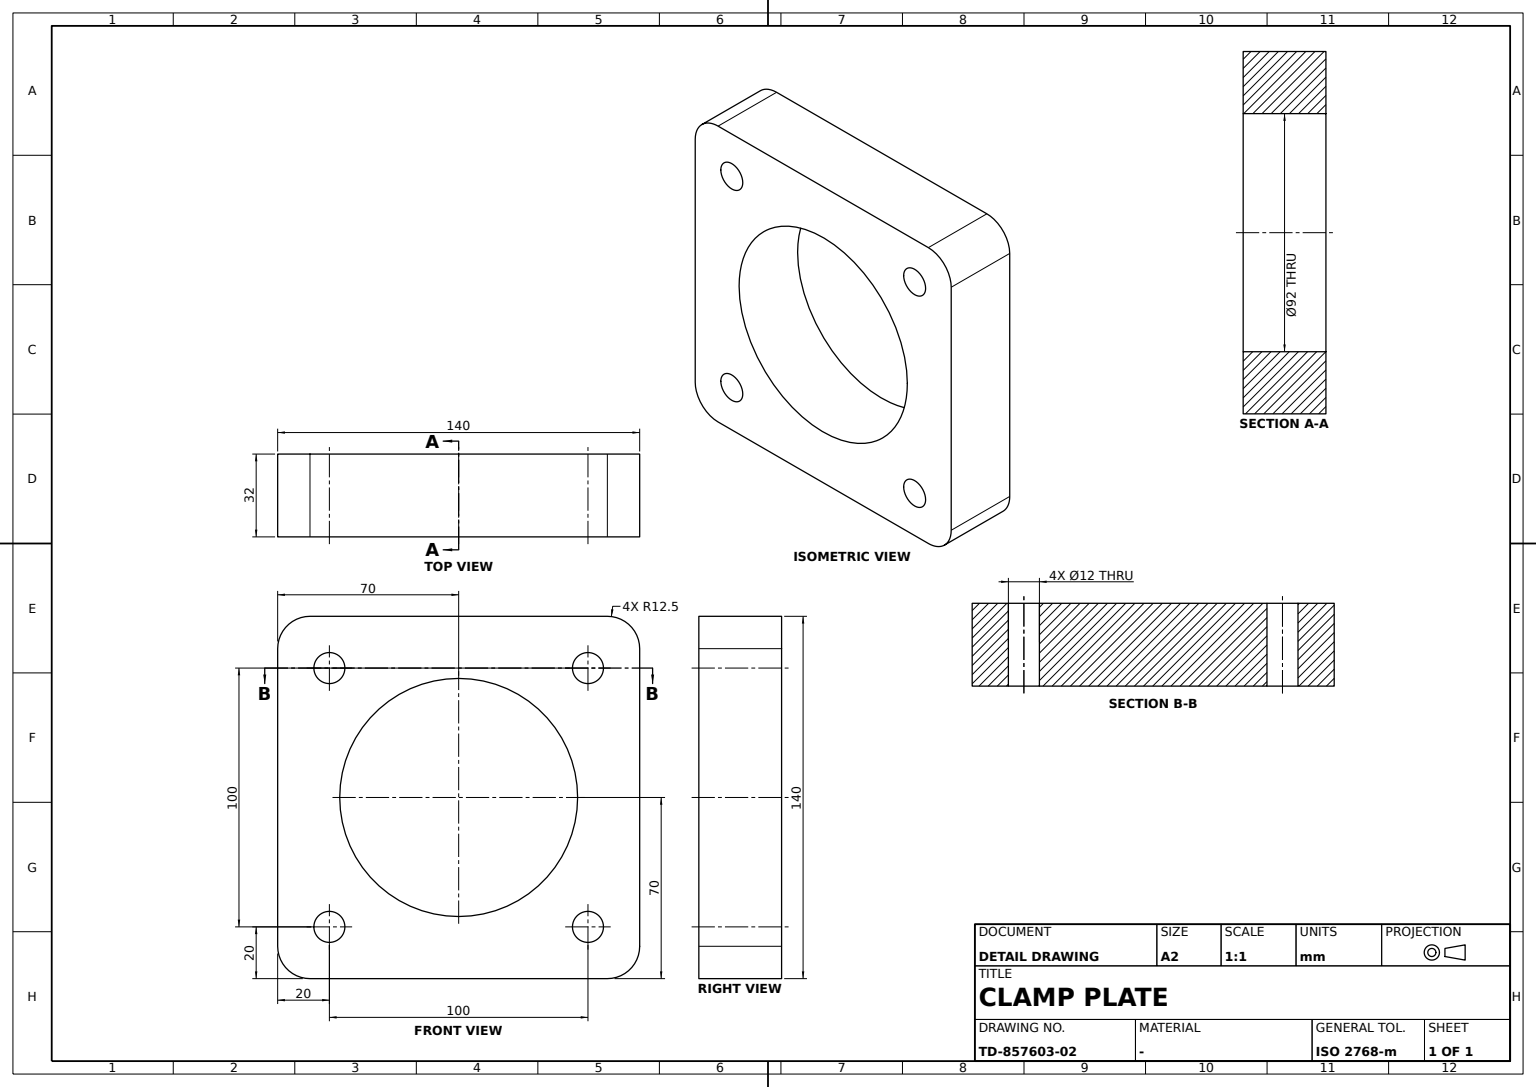
solid
v1 (132.5,-32,28)
v2 (132.5,-32,0)
e1 v1 v2 LINE
v3 (132.5,-60,28)
e2 v1 v3 CIRCLE(AX(P(132.5,-46,28),D(0,0,1),D(1,0,0)),14)
v4 (132.5,-60,0)
e3 v3 v4 LINE
e4 v2 v4 CIRCLE(AX(P(132.5,-46,0),D(0,0,1),D(1,0,0)),14)
face CYL(AX(P(132.5,-46,28),D(0,0,-1),D(1,0,0)),14) rev [-e1 e2 e3 -e4]
v5 (152.5,-89,28)
v6 (152.5,-76.5,28)
e5 v5 v6 LINE
v7 (140,-89,28)
e6 v7 v5 LINE
e7 v6 v7 CIRCLE(AX(P(140,-76.5,28),D(0,0,-1),D(1,0,0)),12.5)
face PLANE(AX(P(0,0,28),D(0,0,1),D(1,0,0))) rev [-e5 -e6 -e7]
v8 (152.5,89,28)
v9 (152.5,89,56)
e8 v8 v9 LINE
v10 (140,89,28)
e9 v8 v10 LINE
v11 (140,89,0)
e10 v11 v10 LINE
v12 (-140,89,0)
e11 v11 v12 LINE
v13 (-140,89,28)
e12 v12 v13 LINE
v14 (-152.5,89,28)
e13 v13 v14 LINE
v15 (-152.5,89,56)
e14 v14 v15 LINE
e15 v9 v15 LINE
face PLANE(AX(P(-152.5,89,0),D(0,-1,0),D(1,0,0))) rev [-e8 e9 -e10 e11 e12 e13 e14 -e15]
v16 (9.365911,-50,0)
v17 (-2.634089,-50,0)
e16 v16 v17 CIRCLE(AX(P(3.365911,-50,0),D(0,0,-1),D(1,0,0)),6)
e17 v17 v16 CIRCLE(AX(P(3.365911,-50,0),D(0,0,-1),D(1,0,0)),6)
face PLANE(AX(P(0,0,0),D(0,0,1),D(1,0,0))) rev [e16 e17]
v18 (-152.5,76.5,28)
e18 v18 v13 CIRCLE(AX(P(-140,76.5,28),D(0,0,-1),D(1,0,0)),12.5)
v19 (-152.5,76.5,0)
e19 v12 v19 CIRCLE(AX(P(-140,76.5,0),D(0,0,1),D(1,0,0)),12.5)
e20 v19 v18 LINE
face CYL(AX(P(-140,76.5,14),D(0,0,-1),D(-1,0,0)),12.5) [e18 -e12 e19 e20]
v20 (152.5,-32,28)
v21 (152.5,-32,0)
e21 v20 v21 LINE
e22 v20 v1 LINE
e23 v21 v2 LINE
face PLANE(AX(P(152.5,-32,28),D(0,1,0),D(1,0,0))) rev [-e21 e22 e1 -e23]
v22 (152.5,-76.5,0)
e24 v22 v6 LINE
v23 (140,-89,0)
e25 v23 v7 LINE
e26 v23 v22 CIRCLE(AX(P(140,-76.5,0),D(0,0,1),D(1,0,0)),12.5)
face CYL(AX(P(140,-76.5,14),D(0,0,-1),D(1,0,0)),12.5) [e24 e7 -e25 e26]
v24 (-2.634089,50,0)
v25 (-2.634089,50,-32)
e27 v24 v25 LINE
v26 (9.365911,50,0)
e28 v26 v24 CIRCLE(AX(P(3.365911,50,0),D(0,0,-1),D(1,0,0)),6)
v27 (9.365911,50,-32)
e29 v26 v27 LINE
e30 v27 v25 CIRCLE(AX(P(3.365911,50,-32),D(0,0,-1),D(1,0,0)),6)
face CYL(AX(P(3.365911,50,-16),D(0,0,1),D(1,0,0)),6) rev [-e27 -e28 e29 e30]
v28 (-2.634089,-50,-32)
v29 (9.365911,-50,-32)
e31 v28 v29 CIRCLE(AX(P(3.365911,-50,-32),D(0,0,-1),D(1,0,0)),6)
e32 v16 v29 LINE
e33 v17 v28 LINE
face CYL(AX(P(3.365911,-50,-16),D(0,0,1),D(1,0,0)),6) rev [e31 -e32 -e17 e33]
v30 (-90.634089,50,0)
v31 (-90.634089,50,-32)
e34 v30 v31 LINE
v32 (-102.634089,50,0)
e35 v32 v30 CIRCLE(AX(P(-96.634089,50,0),D(0,0,-1),D(1,0,0)),6)
v33 (-102.634089,50,-32)
e36 v32 v33 LINE
e37 v33 v31 CIRCLE(AX(P(-96.634089,50,-32),D(0,0,-1),D(1,0,0)),6)
face CYL(AX(P(-96.634089,50,-16),D(0,0,1),D(1,0,0)),6) rev [-e34 -e35 e36 e37]
v34 (-116.634089,57.5,0)
v35 (-116.634089,57.5,-32)
e38 v34 v35 LINE
v36 (-116.634089,-57.5,-32)
e39 v36 v35 LINE
v37 (-116.634089,-57.5,0)
e40 v37 v36 LINE
e41 v37 v34 LINE
face PLANE(AX(P(-116.634089,-70,0),D(-1,0,0),D(0,1,0))) [e38 -e39 -e40 e41]
v38 (-102.634089,-50,0)
v39 (-90.634089,-50,0)
e42 v38 v39 CIRCLE(AX(P(-96.634089,-50,0),D(0,0,-1),D(1,0,0)),6)
v40 (-102.634089,-50,-32)
e43 v38 v40 LINE
v41 (-90.634089,-50,-32)
e44 v40 v41 CIRCLE(AX(P(-96.634089,-50,-32),D(0,0,-1),D(1,0,0)),6)
e45 v39 v41 LINE
face CYL(AX(P(-96.634089,-50,-16),D(0,0,1),D(1,0,0)),6) rev [-e42 e43 e44 -e45]
v42 (23.365911,-57.5,0)
v43 (10.865911,-70,0)
e46 v42 v43 CIRCLE(AX(P(10.865911,-57.5,0),D(0,0,-1),D(1,0,0)),12.5)
v44 (10.865911,-70,-32)
e47 v43 v44 LINE
v45 (23.365911,-57.5,-32)
e48 v44 v45 CIRCLE(AX(P(10.865911,-57.5,-32),D(0,0,1),D(1,0,0)),12.5)
e49 v42 v45 LINE
face CYL(AX(P(10.865911,-57.5,-16),D(0,0,1),D(0,-1,0)),12.5) [e46 e47 e48 -e49]
v46 (-132.5,32,28)
v47 (-118.5,46,28)
e50 v46 v47 CIRCLE(AX(P(-132.5,46,28),D(0,0,1),D(1,0,0)),14)
v48 (-152.5,32,28)
e51 v48 v46 LINE
v49 (-152.5,60,28)
e52 v49 v48 LINE
v50 (-132.5,60,28)
e53 v49 v50 LINE
e54 v47 v50 CIRCLE(AX(P(-132.5,46,28),D(0,0,1),D(1,0,0)),14)
face PLANE(AX(P(0,0,28),D(0,0,1),D(1,0,0))) rev [-e50 -e51 -e52 e53 -e54]
v51 (-118.5,-46,0)
v52 (-132.5,-32,0)
e55 v51 v52 CIRCLE(AX(P(-132.5,-46,0),D(0,0,1),D(1,0,0)),14)
v53 (-118.5,-46,28)
e56 v53 v51 LINE
v54 (-132.5,-32,28)
e57 v53 v54 CIRCLE(AX(P(-132.5,-46,28),D(0,0,1),D(1,0,0)),14)
e58 v54 v52 LINE
face CYL(AX(P(-132.5,-46,28),D(0,0,-1),D(1,0,0)),14) rev [-e55 -e56 e57 e58]
v55 (-152.5,-32,28)
v56 (-152.5,-32,0)
e59 v55 v56 LINE
e60 v52 v56 LINE
e61 v55 v54 LINE
face PLANE(AX(P(152.5,-32,28),D(0,1,0),D(1,0,0))) rev [e59 -e60 -e58 -e61]
e62 v30 v32 CIRCLE(AX(P(-96.634089,50,0),D(0,0,-1),D(1,0,0)),6)
face PLANE(AX(P(0,0,0),D(0,0,1),D(1,0,0))) rev [e62 e35]
e63 v25 v27 CIRCLE(AX(P(3.365911,50,-32),D(0,0,-1),D(1,0,0)),6)
e64 v24 v26 CIRCLE(AX(P(3.365911,50,0),D(0,0,-1),D(1,0,0)),6)
face CYL(AX(P(3.365911,50,-16),D(0,0,1),D(1,0,0)),6) rev [e63 -e29 -e64 e27]
e65 v31 v33 CIRCLE(AX(P(-96.634089,50,-32),D(0,0,-1),D(1,0,0)),6)
face CYL(AX(P(-96.634089,50,-16),D(0,0,1),D(1,0,0)),6) rev [e65 -e36 -e62 e34]
v57 (23.365911,57.5,-32)
e66 v57 v45 LINE
v58 (23.365911,57.5,0)
e67 v58 v57 LINE
e68 v58 v42 LINE
face PLANE(AX(P(23.365911,70,0),D(1,0,0),D(0,-1,0))) [-e66 -e67 e68 e49]
e69 v39 v38 CIRCLE(AX(P(-96.634089,-50,0),D(0,0,-1),D(1,0,0)),6)
face PLANE(AX(P(0,0,0),D(0,0,1),D(1,0,0))) rev [e69 e42]
v59 (-118.5,46,0)
v60 (-132.5,60,0)
e70 v59 v60 CIRCLE(AX(P(-132.5,46,0),D(0,0,1),D(1,0,0)),14)
e71 v47 v59 LINE
e72 v50 v60 LINE
face CYL(AX(P(-132.5,46,28),D(0,0,-1),D(1,0,0)),14) rev [-e70 -e71 e54 e72]
v61 (132.5,58.059115,28)
v62 (132.5,58.059115,0)
e73 v61 v62 LINE
v63 (132.5,33.940885,28)
e74 v61 v63 CIRCLE(AX(P(132.5,46,28),D(0,0,1),D(1,0,0)),12.059115)
v64 (132.5,33.940885,0)
e75 v63 v64 LINE
e76 v62 v64 CIRCLE(AX(P(132.5,46,0),D(0,0,1),D(1,0,0)),12.059115)
face CYL(AX(P(132.5,46,20),D(0,0,-1),D(1,0,0)),12.059115) rev [-e73 e74 e75 -e76]
v65 (152.5,58.059115,0)
e77 v65 v62 LINE
v66 (152.5,58.059115,28)
e78 v66 v65 LINE
e79 v66 v61 LINE
face PLANE(AX(P(152.5,58.059115,20),D(0,1,0),D(1,0,0))) rev [-e77 -e78 e79 e73]
v67 (-140,-89,28)
v68 (-152.5,-76.5,28)
e80 v67 v68 CIRCLE(AX(P(-140,-76.5,28),D(0,0,-1),D(1,0,0)),12.5)
v69 (-152.5,-76.5,0)
e81 v69 v68 LINE
v70 (-140,-89,0)
e82 v69 v70 CIRCLE(AX(P(-140,-76.5,0),D(0,0,1),D(1,0,0)),12.5)
e83 v70 v67 LINE
face CYL(AX(P(-140,-76.5,14),D(0,0,-1),D(0,-1,0)),12.5) [e80 -e81 e82 e83]
e84 v14 v18 LINE
face PLANE(AX(P(0,0,28),D(0,0,1),D(1,0,0))) rev [-e84 -e13 -e18]
v71 (-152.5,-89,28)
e85 v71 v67 LINE
e86 v68 v71 LINE
face PLANE(AX(P(0,0,28),D(0,0,1),D(1,0,0))) rev [-e80 -e85 -e86]
v72 (-152.5,-89,56)
e87 v71 v72 LINE
e88 v15 v72 LINE
v73 (-152.5,60,0)
e89 v19 v73 LINE
e90 v49 v73 LINE
v74 (-152.5,32,0)
e91 v48 v74 LINE
e92 v74 v56 LINE
v75 (-152.5,-60,28)
e93 v55 v75 LINE
v76 (-152.5,-60,0)
e94 v75 v76 LINE
e95 v76 v69 LINE
face PLANE(AX(P(-152.5,89,0),D(-1,0,0),D(0,-1,0))) [e86 e87 -e88 -e14 e84 -e20 e89 -e90 e52 e91 e92 -e59 e93 e94 e95 e81]
v77 (-132.5,-60,0)
e96 v77 v51 CIRCLE(AX(P(-132.5,-46,0),D(0,0,1),D(1,0,0)),14)
v78 (-132.5,-60,28)
e97 v78 v77 LINE
e98 v78 v53 CIRCLE(AX(P(-132.5,-46,28),D(0,0,1),D(1,0,0)),14)
face CYL(AX(P(-132.5,-46,28),D(0,0,-1),D(1,0,0)),14) rev [-e96 -e97 e98 e56]
e99 v70 v23 LINE
v79 (152.5,-89,56)
e100 v5 v79 LINE
e101 v72 v79 LINE
face PLANE(AX(P(152.5,-89,0),D(0,1,0),D(-1,0,0))) rev [e99 e25 e6 e100 -e101 -e87 e85 -e83]
v80 (152.5,-60,28)
e102 v80 v20 LINE
e103 v80 v3 LINE
face PLANE(AX(P(0,0,28),D(0,0,1),D(1,0,0))) rev [-e2 -e22 -e102 e103]
e104 v75 v78 LINE
face PLANE(AX(P(0,0,28),D(0,0,1),D(1,0,0))) rev [-e93 e61 -e57 -e98 -e104]
e105 v79 v9 LINE
face PLANE(AX(P(0,0,56),D(0,0,1),D(1,0,0))) [e15 e88 e101 e105]
e106 v60 v73 LINE
face PLANE(AX(P(-132.5,60,28),D(0,-1,0),D(-1,0,0))) [e90 -e106 -e72 -e53]
v81 (152.5,76.5,0)
e107 v81 v11 CIRCLE(AX(P(140,76.5,0),D(0,0,1),D(1,0,0)),12.5)
e108 v65 v81 LINE
v82 (152.5,33.940885,0)
e109 v82 v64 LINE
e110 v21 v82 LINE
v83 (152.5,-60,0)
e111 v4 v83 LINE
e112 v22 v83 LINE
e113 v76 v77 LINE
v84 (-132.5,32,0)
e114 v74 v84 LINE
e115 v84 v59 CIRCLE(AX(P(-132.5,46,0),D(0,0,1),D(1,0,0)),14)
v85 (-104.134089,-70,0)
e116 v43 v85 LINE
v86 (10.865911,70,0)
e117 v86 v58 CIRCLE(AX(P(10.865911,57.5,0),D(0,0,-1),D(1,0,0)),12.5)
v87 (-104.134089,70,0)
e118 v87 v86 LINE
e119 v34 v87 CIRCLE(AX(P(-104.134089,57.5,0),D(0,0,-1),D(1,0,0)),12.5)
e120 v85 v37 CIRCLE(AX(P(-104.134089,-57.5,0),D(0,0,-1),D(1,0,0)),12.5)
face PLANE(AX(P(0,0,0),D(0,0,1),D(1,0,0))) rev [-e11 -e107 -e108 e77 e76 -e109 -e110 e23 e4 e111 -e112 -e26 -e99 -e82 -e95 e113 e96 e55 e60 -e92 e114 e115 e70 e106 -e89 -e19] [-e116 -e46 -e68 -e117 -e118 -e119 -e41 -e120]
v88 (152.5,76.5,28)
e121 v88 v8 LINE
e122 v10 v88 CIRCLE(AX(P(140,76.5,28),D(0,0,-1),D(1,0,0)),12.5)
face PLANE(AX(P(0,0,28),D(0,0,1),D(1,0,0))) rev [-e9 -e121 -e122]
e123 v29 v28 CIRCLE(AX(P(3.365911,-50,-32),D(0,0,-1),D(1,0,0)),6)
face CYL(AX(P(3.365911,-50,-16),D(0,0,1),D(1,0,0)),6) rev [e32 e123 -e33 -e16]
v89 (152.5,33.940885,28)
e124 v89 v66 LINE
e125 v89 v63 LINE
face PLANE(AX(P(0,0,28),D(0,0,1),D(1,0,0))) rev [-e124 e125 -e74 -e79]
e126 v41 v40 CIRCLE(AX(P(-96.634089,-50,-32),D(0,0,-1),D(1,0,0)),6)
face CYL(AX(P(-96.634089,-50,-16),D(0,0,1),D(1,0,0)),6) rev [e45 e126 -e43 -e69]
v90 (-104.134089,-70,-32)
e127 v36 v90 CIRCLE(AX(P(-104.134089,-57.5,-32),D(0,0,1),D(1,0,0)),12.5)
e128 v85 v90 LINE
face CYL(AX(P(-104.134089,-57.5,-16),D(0,0,1),D(-1,0,0)),12.5) [e127 -e128 e120 e40]
v91 (-104.134089,70,-32)
e129 v87 v91 LINE
v92 (10.865911,70,-32)
e130 v86 v92 LINE
e131 v91 v92 LINE
face PLANE(AX(P(23.365911,70,0),D(0,-1,0),D(-1,0,0))) rev [-e129 e118 e130 -e131]
e132 v57 v92 CIRCLE(AX(P(10.865911,57.5,-32),D(0,0,1),D(1,0,0)),12.5)
face CYL(AX(P(10.865911,57.5,-16),D(0,0,1),D(1,0,0)),12.5) [e132 -e130 e117 e67]
e133 v81 v88 LINE
face CYL(AX(P(140,76.5,14),D(0,0,-1),D(0,1,0)),12.5) [e122 -e133 e107 e10]
e134 v46 v84 LINE
face PLANE(AX(P(-152.5,32,28),D(0,-1,0),D(-1,0,0))) rev [e134 -e114 -e91 e51]
e135 v80 v83 LINE
face PLANE(AX(P(132.5,-60,28),D(0,1,0),D(1,0,0))) [-e3 -e103 e135 -e111]
e136 v91 v35 CIRCLE(AX(P(-104.134089,57.5,-32),D(0,0,1),D(1,0,0)),12.5)
face CYL(AX(P(-104.134089,57.5,-16),D(0,0,1),D(0,1,0)),12.5) [e119 e129 e136 -e38]
e137 v89 v82 LINE
face PLANE(AX(P(132.5,33.940885,20),D(0,1,0),D(1,0,0))) [-e75 -e125 e137 e109]
e138 v44 v90 LINE
face PLANE(AX(P(-116.634089,-70,0),D(0,1,0),D(1,0,0))) rev [e116 e128 -e138 -e47]
face PLANE(AX(P(0,0,0),D(0,0,1),D(1,0,0))) rev [e28 e64]
face CYL(AX(P(-132.5,46,28),D(0,0,-1),D(1,0,0)),14) rev [-e115 -e134 e50 e71]
face PLANE(AX(P(0,0,-32),D(0,0,-1),D(1,0,0))) [-e37 -e65] [-e127 e39 -e136 e131 -e132 e66 -e48 e138] [-e30 -e63] [-e44 -e126] [-e31 -e123]
face PLANE(AX(P(152.5,-89,0),D(1,0,0),D(0,1,0))) [e8 -e105 -e100 e5 -e24 e112 -e135 e102 e21 e110 -e137 e124 e78 e108 e133 e121]
face PLANE(AX(P(132.5,-60,28),D(0,1,0),D(1,0,0))) [e97 -e113 -e94 e104]
